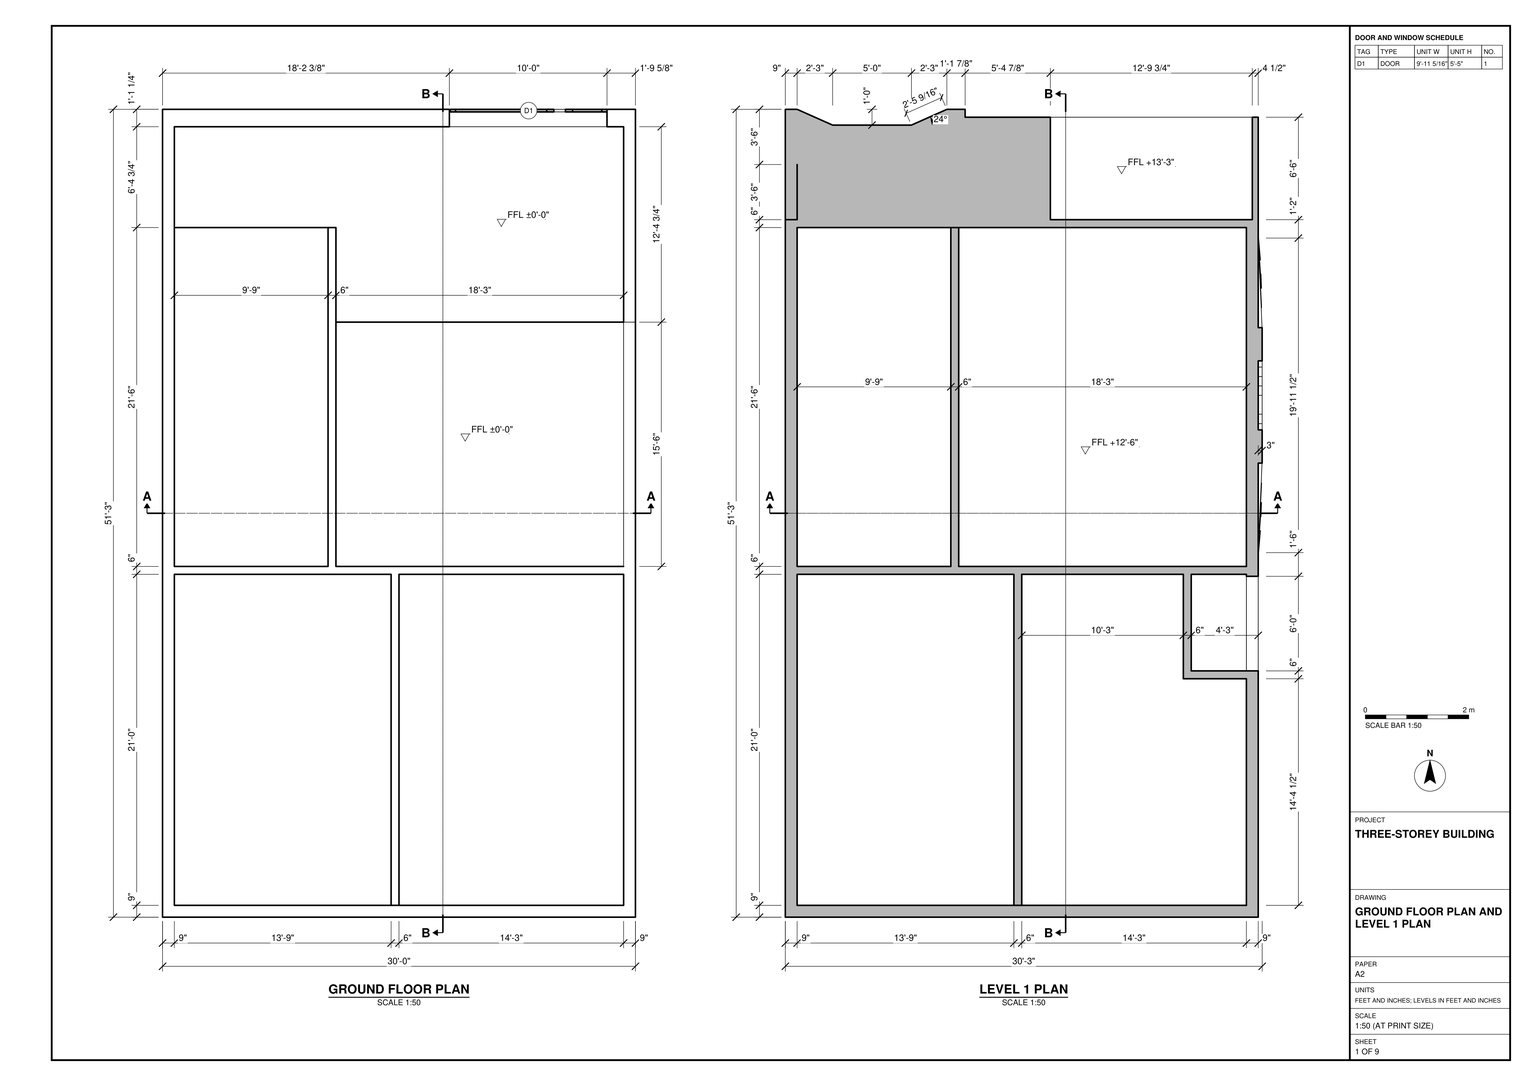
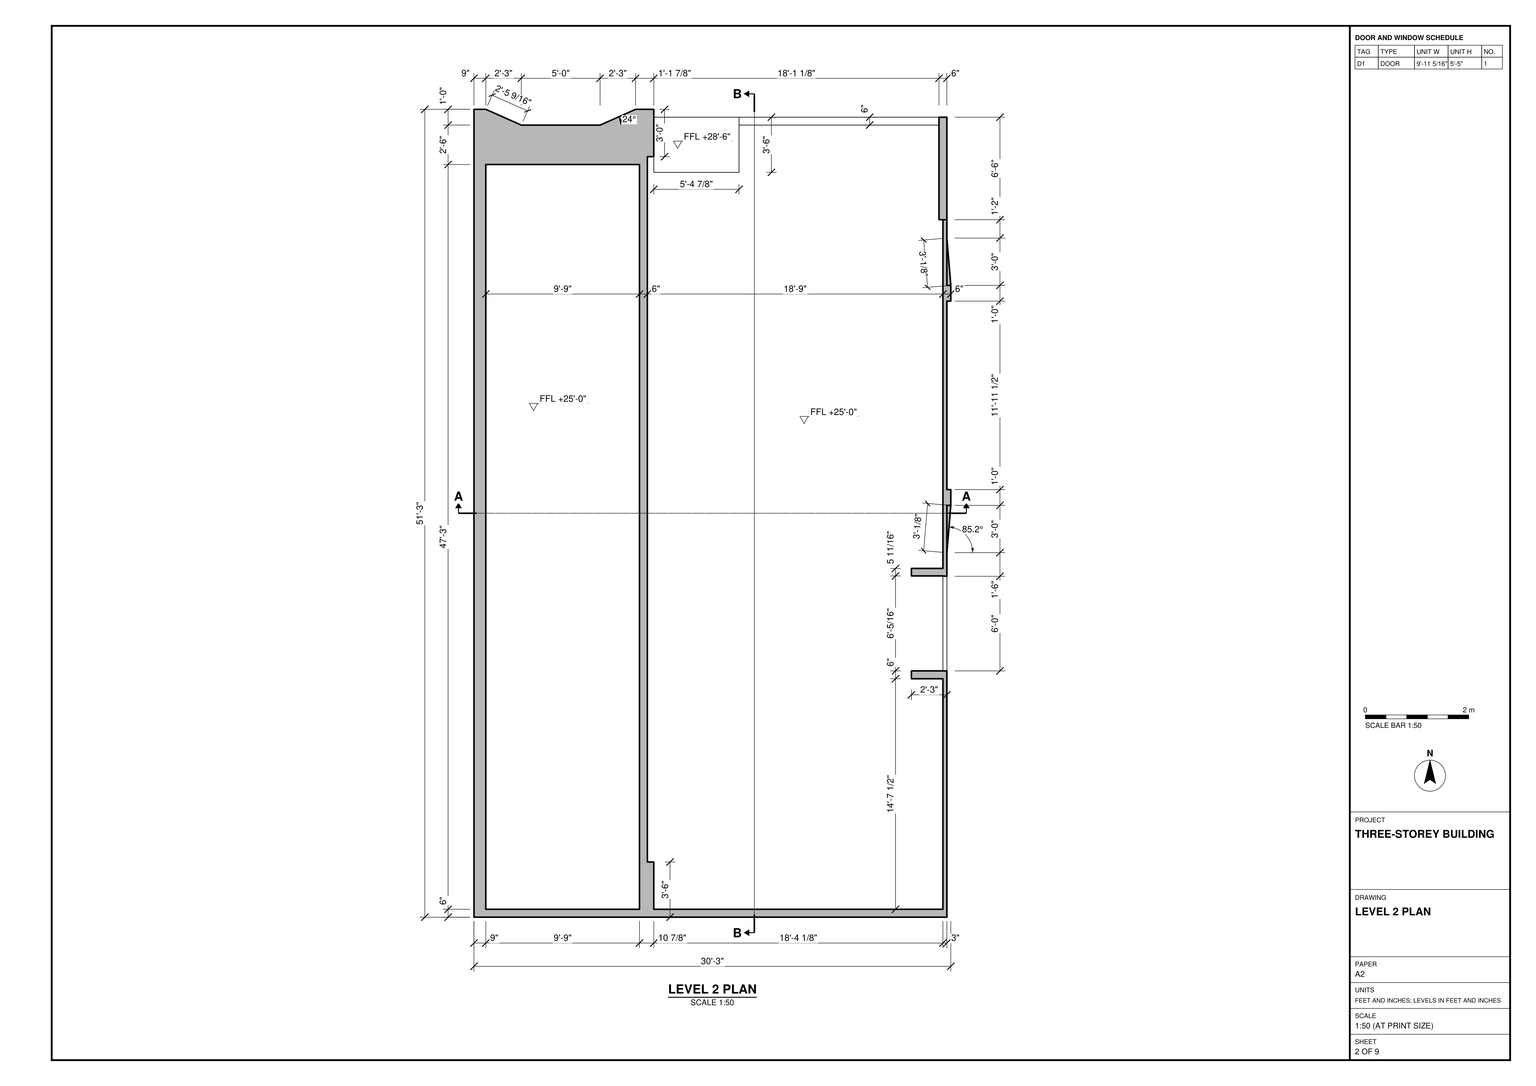
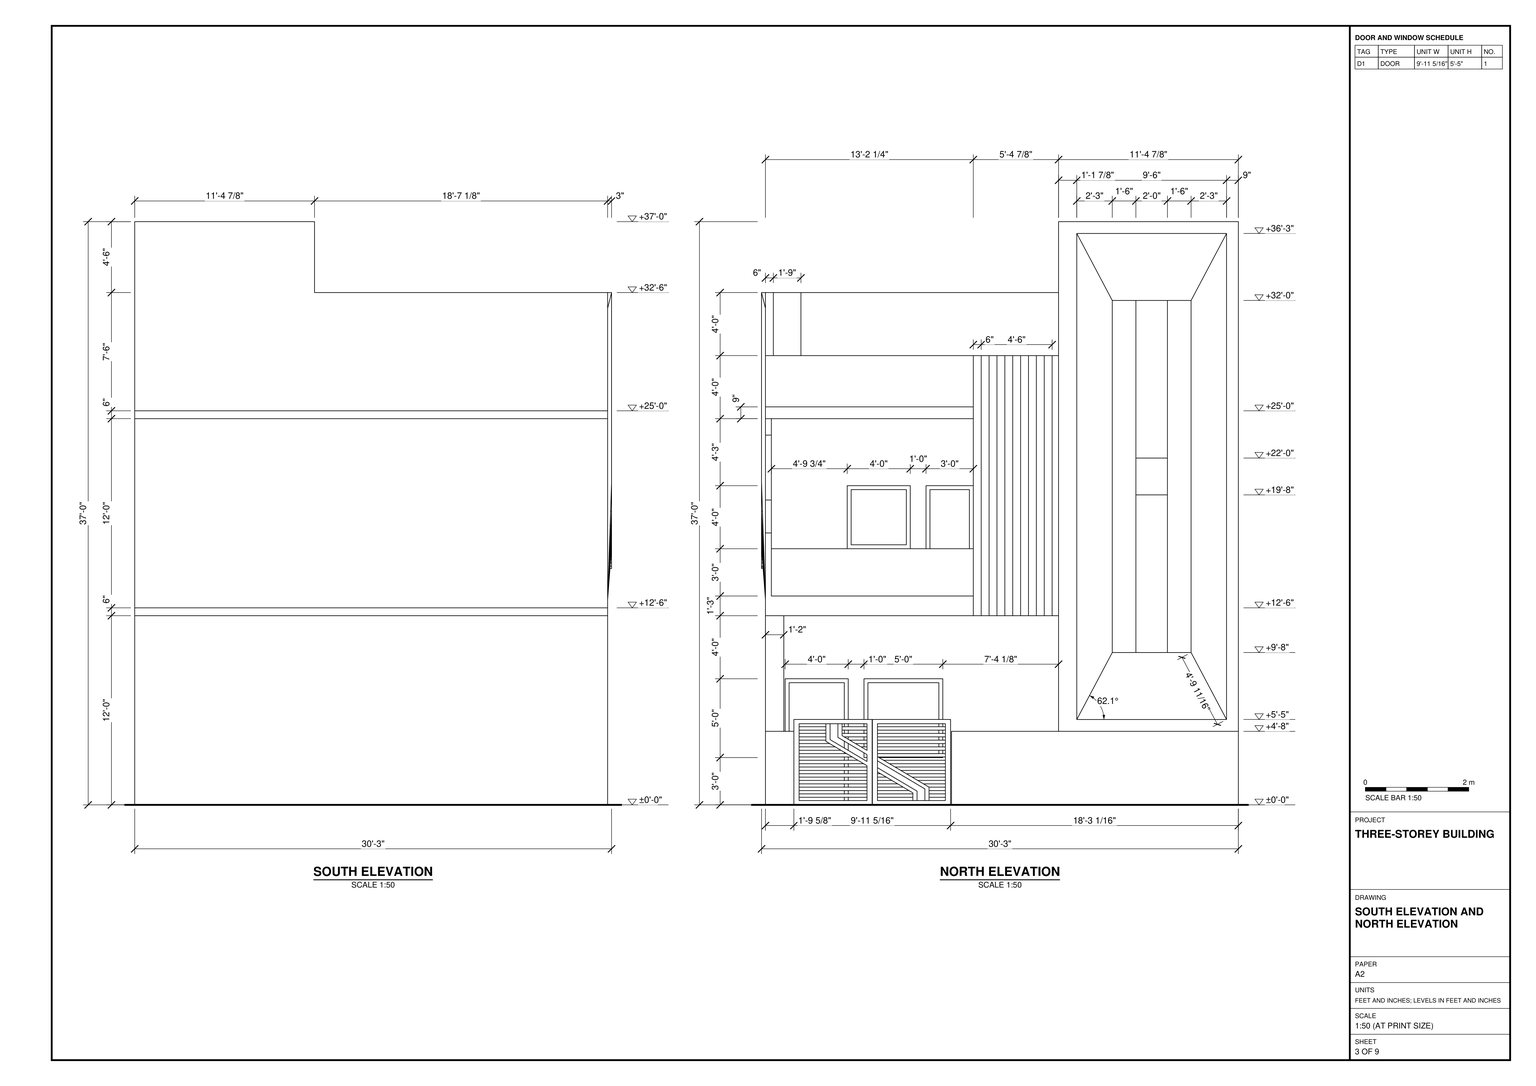
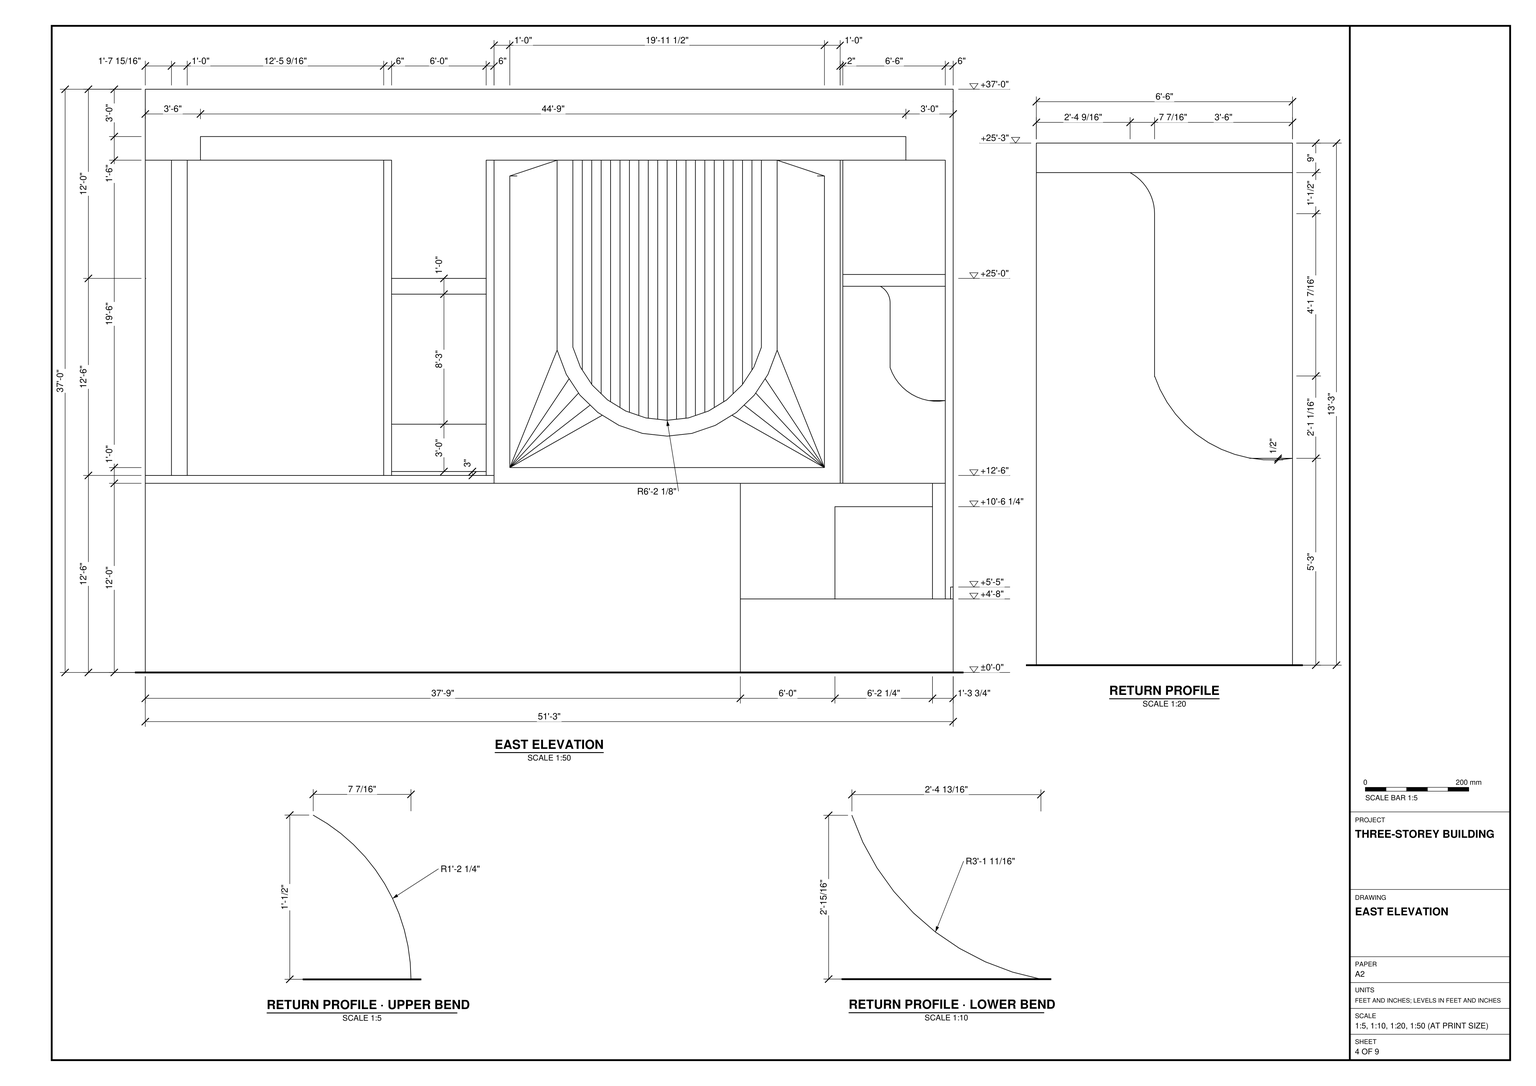
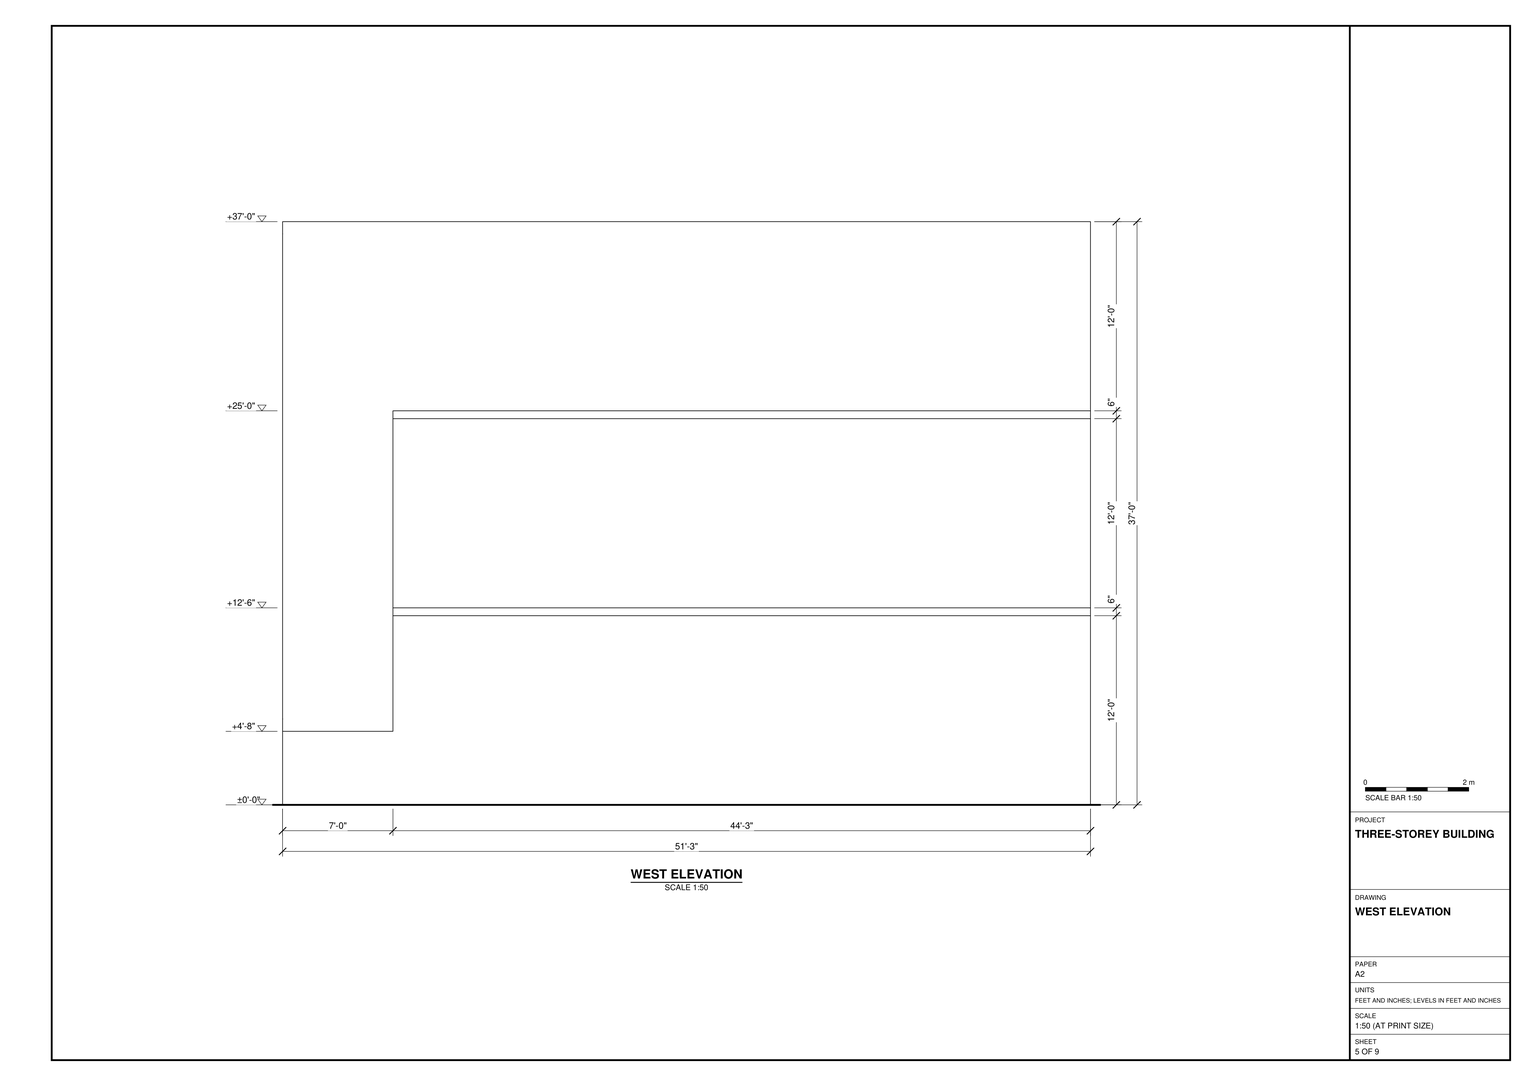
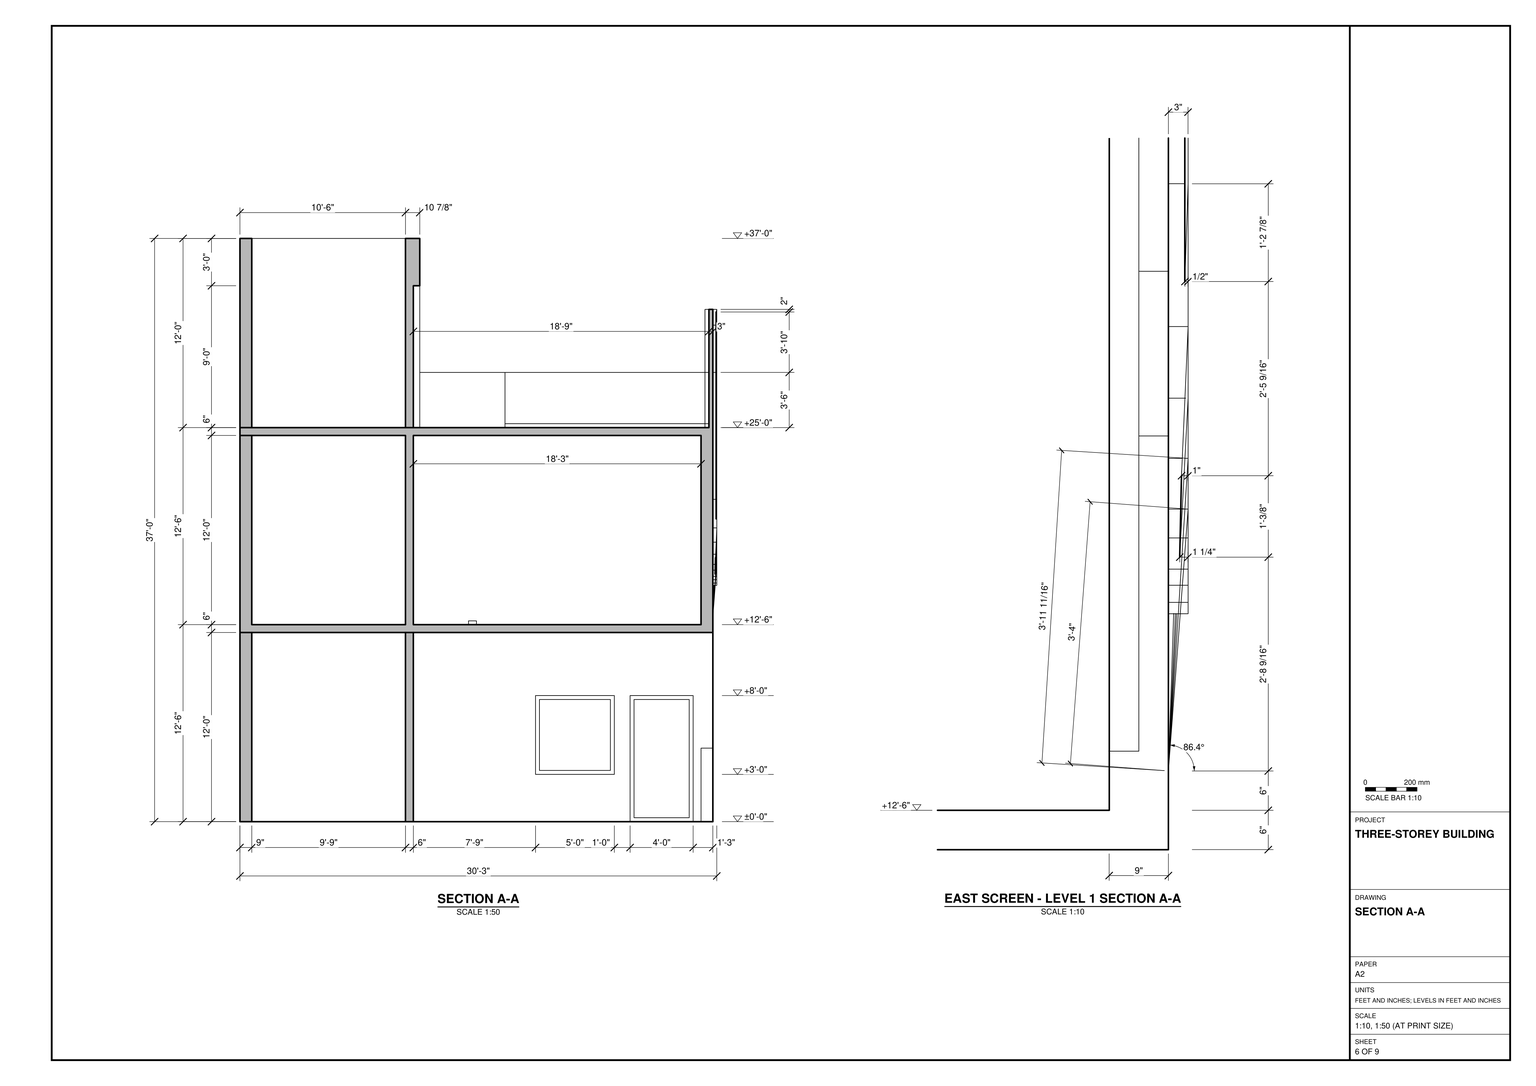
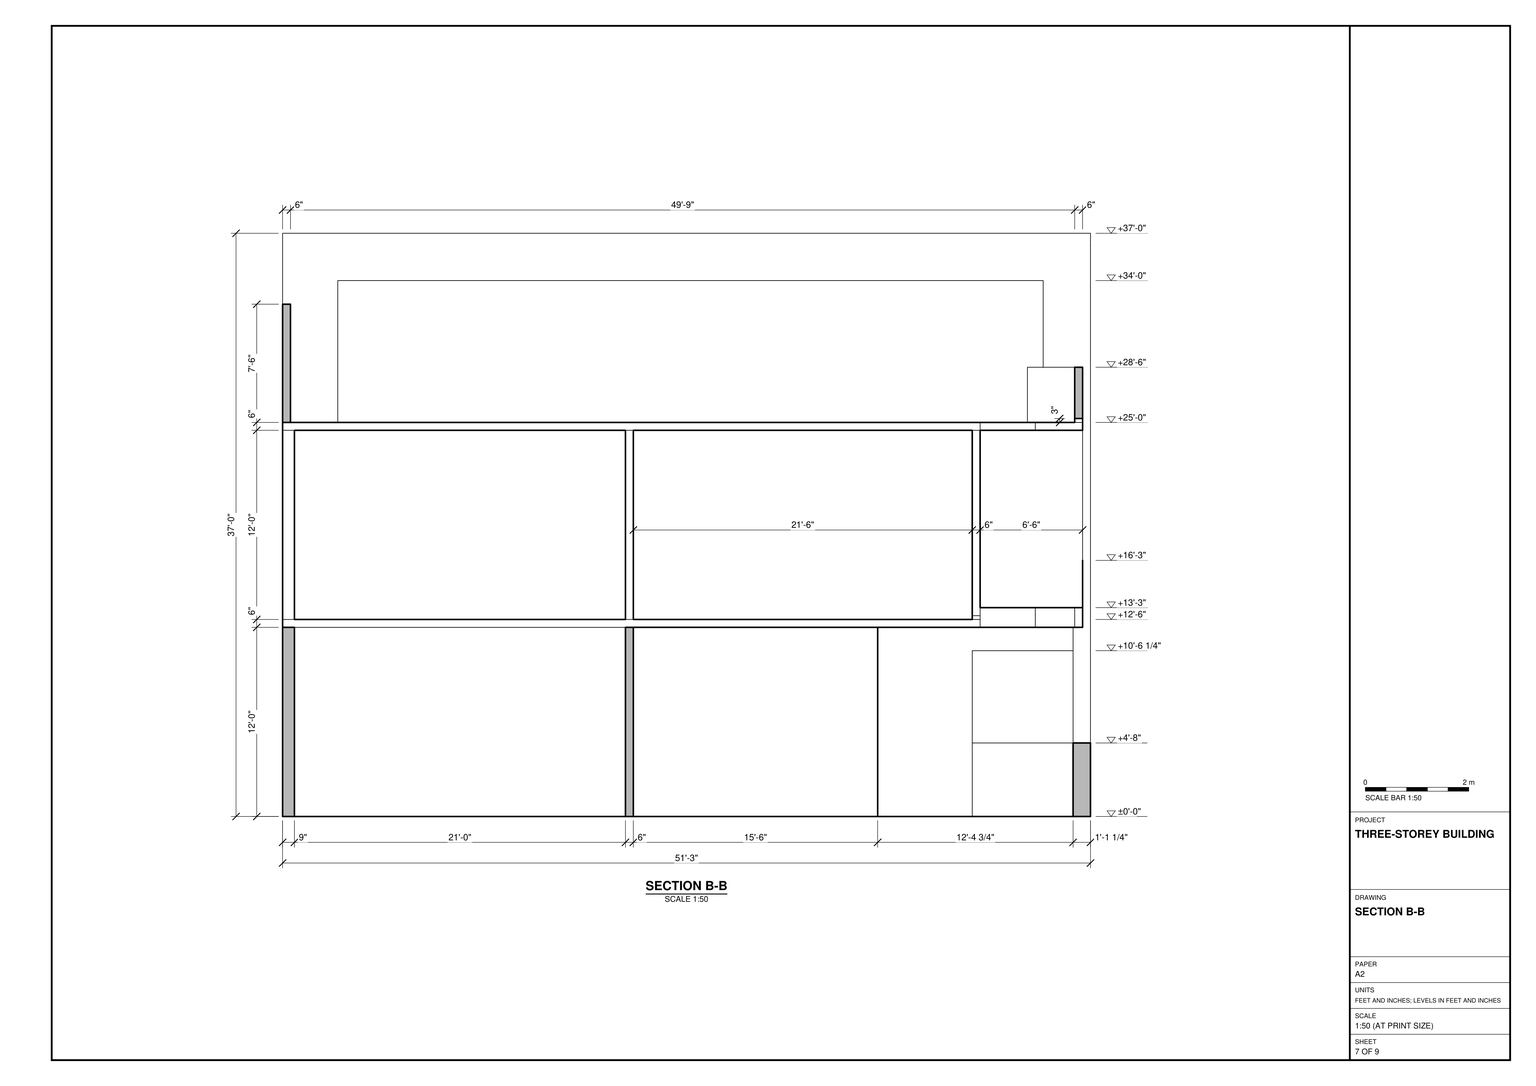
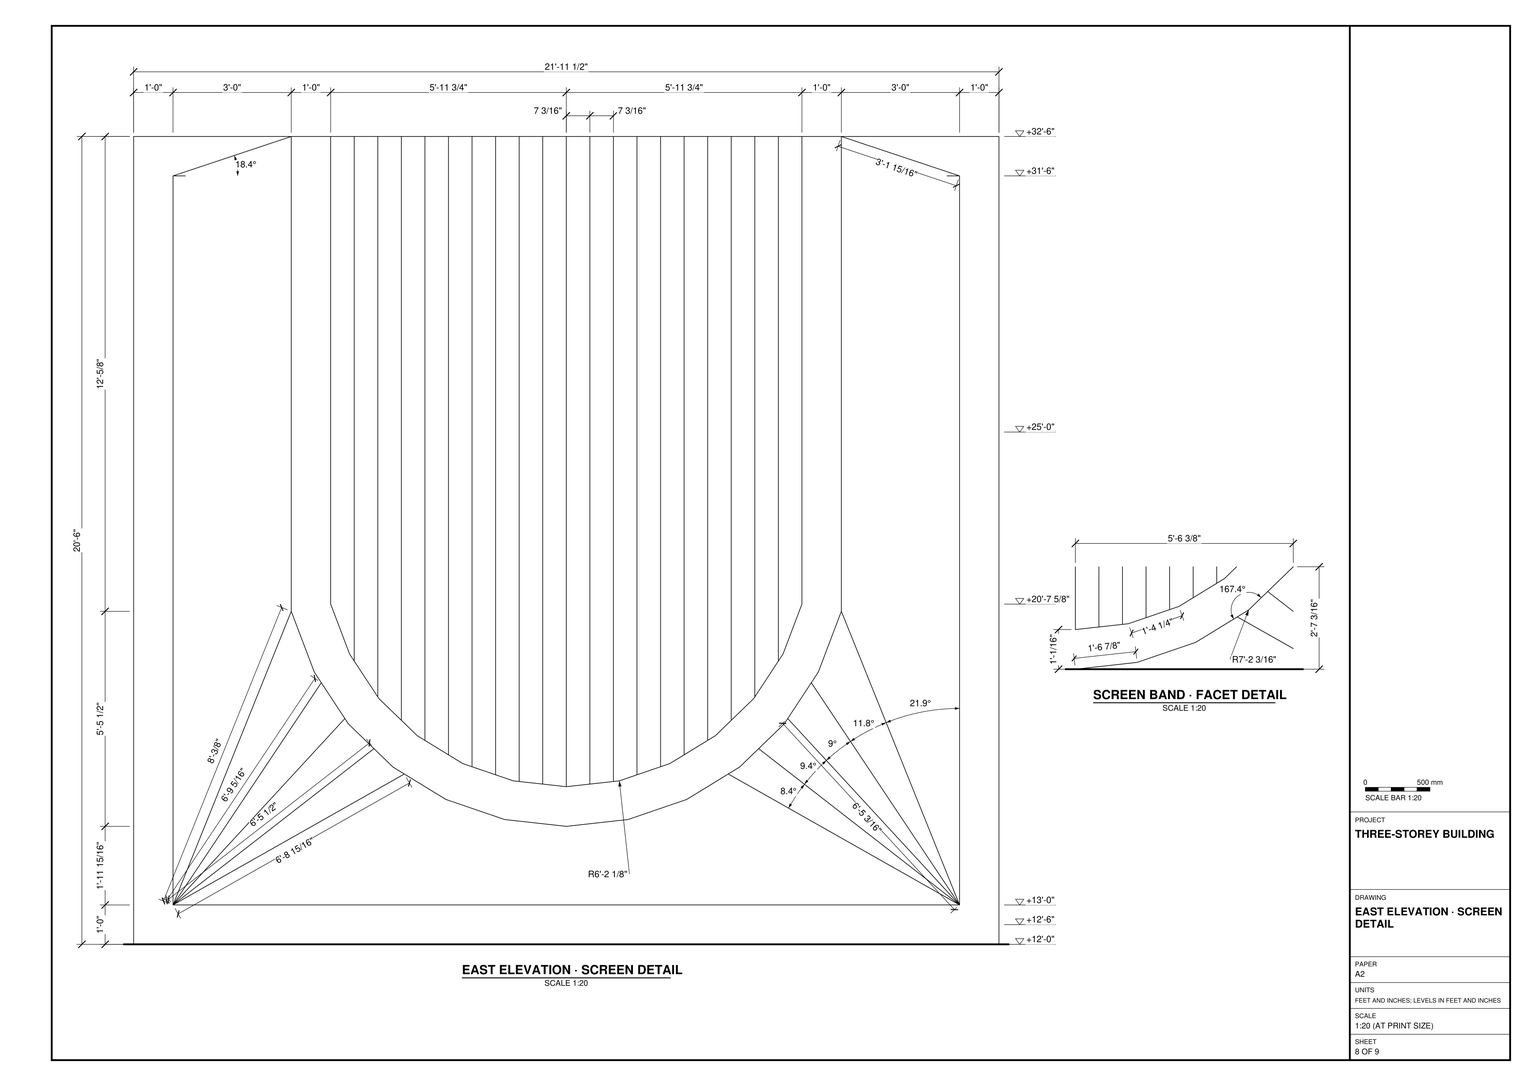
Work in feet and inches to build the three-storey building shown in task_files/diagram_01.pdf. The overall model measures 30'-3" east to west, 51'-3" north to south and 37'-0" high. Set the ground floor at ±0'-0", level 1 at +12'-6" and level 2 at +25'-0".

Use each floor plan separately: the partitions change between storeys. On the ground floor, place the two rear bays side by side and offset their dividing wall from the partition farther north. On level 1, follow the wall return on the east side. On level 2, form the long, narrow western bay beside the wider eastern area. Use the wall thicknesses shown, including the 9" perimeter walls and 6" partitions where indicated. Match the floor slabs and stepped roof edges to the elevations.

On the north frontage, place the two-leaf entrance gate in the low wall and set the window openings behind it. Model the vertical fins and the tall recessed panel with sloping reveals. Keep shell elements such as walls, slabs and roof separate as groups or components. Group each furniture or joinery piece shown separately and use components for repeated parts. Decor and loose items may be any suitable library components. Save one SketchUp model as output_files/three_storey_building_with_a_stepped_roofline.skp.

# SketchUp Ruby script. Lengths in inches.
U = 1.inch
M = Sketchup.active_model
def pt(a) = Geom::Point3d.new(a.map { |v| v * U })
def face(e, loops, mat)
  f = e.add_face(loops[0].map { |a| pt(a) })
  loops[1..].each { |l| e.add_face(l.map { |a| pt(a) }).erase! }
  f.material = f.back_material = mat if mat
  f
end
# faces: each face lists its corners as indices into pts; further lists are holes
def faces(e, pts, list, mat = nil) = list.each { |f| face(e, (f[0].is_a?(Array) ? f : [f]).map { |l| l.map { |i| pts[i] } }, mat) }
# xy, xz, yz: faces in a plane at the given z, y or x. An outline is a flat list of corners, or four numbers for a rectangle; further outlines are holes
def ring(l) = l.size == 4 ? [[l[0], l[1]], [l[2], l[1]], [l[2], l[3]], [l[0], l[3]]] : l.each_slice(2).to_a
def flat(e, list, mat, &to3) = list.each { |f| face(e, (f[0].is_a?(Array) ? f : [f]).map { |l| ring(l).map { |u, v| to3.(u, v) } }, mat) }
def xy(e, z, list, mat = nil) = flat(e, list, mat) { |x, y| [x, y, z] }
def xz(e, y, list, mat = nil) = flat(e, list, mat) { |x, z| [x, y, z] }
def yz(e, x, list, mat = nil) = flat(e, list, mat) { |y, z| [x, y, z] }
def lines(e, pts, list) = list.each { |a, b| e.add_line(pt(pts[a]), pt(pts[b])) }
# prism: a flat outline (further loops are holes) pulled along v
def prism(e, loops, v, mat = nil)
  f = face(e, loops, mat); d = Geom::Vector3d.new(v.map { |x| x * U })
  f.pushpull(f.normal.samedirection?(d) ? d.length : -d.length)
end
def box(e, o, s, mat = nil) = prism(e, [[o, [o[0] + s[0], o[1], o[2]], [o[0] + s[0], o[1] + s[1], o[2]], [o[0], o[1] + s[1], o[2]]]], [0, 0, s[2]], mat)
def at(x, y, z, deg = 0) = Geom::Transformation.translation(pt([x, y, z])) * Geom::Transformation.rotation(ORIGIN, Z_AXIS, deg.degrees)
def axes(o, x, y, z) = Geom::Transformation.new([*x, 0, *y, 0, *z, 0, *pt(o).to_a, 1])
def part(name) = M.definitions.add(name)
# library, detail: a bought-in or finely detailed component or shape, given as its bounding box
def library(name, o, s) = part(name).tap { |d| box(d.entities, o, s) }
def detail(e, o, s) = box(e.add_group.entities, o, s)
def put(e, d, t, mat = nil) = e.add_instance(d, t).tap { |i| i.material = mat if mat }
def group(e, t, mat = nil) = e.add_group.tap { |g| g.transformation = t; g.material = mat if mat }.entities
root = M.entities
M.materials.add("B03_Apricot_Glow").color = [255, 140, 101]
M.materials.add("Carpet_2_1K").color = [173, 65, 48]
M.materials.add("Crushed_Rock_Gravel_1K").color = [234, 234, 234]
M.materials.add("Glass_Basic_01").color = [149, 186, 85]
M.materials["Glass_Basic_01"].alpha = 0.25
M.materials.add("Glass_Mirror_01").color = [185, 185, 185]
M.materials.add("ThomThom - Trousers1").color = [162, 168, 168]
M.materials.add("ThomThom - Waistcoat2").color = [127, 127, 126]
M.materials.add("Wood_Veneer_15_1K").color = [103, 69, 45]
c1 = library("Modern+Gate+1",[0,0,0],[118.11,1.97,78.74])
xy(root,0,[[[0,0,360,0,360,453,351,453,351,267,132,267,132,525,126,525,126,267,9,267,9,601.76,218.36,601.76,218.36,615,0,615],[180,9,351,261],[9,9,174,261]],[9,9,174,261],[180,9,351,261],[9,267,126,525],[132,267,351,453],
  [132,453,351,453,351,601.76,9,601.76,9,525,132,525],[351,453,360,453,360,615,338.36,615,338.36,601.76,351,601.76],[218.36,601.76,338.36,615]])
xy(root,55.98,[[351,453,360,599.24],[346.02,599.24,351,601.76],[351,599.24,351,601.76,346.02,601.76,346.02,609,360,609,360,599.24],[136.89,601.76,218.36,615],[338.36,601.76,346.02,601.76,346.02,609,360,609,360,615,338.36,615]])
xy(root,126.22,[[126,525,132,601.76]])
xy(root,144,[[0,0,9,531],[[9,0,9,9,174,9,174,261,132,261,132,267,351,267,351,453,360,453,360,0],[180,9,351,261]],[[9,9,9,525,126,525,126,601.76,132,601.76,132,453,351,453,351,267,132,267,132,261,174,261,174,9],[126,348,132,354]],[9,261,132,261,132,348,126,348,126,267,9,267],[126,348,132,354],
  [126,354,132,601.76],[9,525,126,601.76],[346.02,599.24,360,609]])
xy(root,144,[[132,453,132,601.76,136.89,601.76,136.89,609,346.02,609,346.02,599.24,360,599.24,360,453]],"Wood_Veneer_15_1K")
xy(root,150,[[9,9,174,261],[180,9,351,9,351,181.5,303,181.5,303,261,180,261],[309,187.5,351,261],[9,267,126,525],[132,267,351,525]])
xy(root,153,[[351,187.5,360,259.5]])
xy(root,159,[[201.77,531,355.5,609]])
xy(root,207,[[355.5,596.6875,360,609]])
xy(root,288,[[303,181.5,351,181.5,351,187.5,309,187.5,309,261,303,261],[351,187.5,360,259.5]])
xy(root,294,[[0,0,0,531,9,531,9,525,351,525,351,267,132,267,132,525,126,525,126,267,9,267,9,261,174,261,174,9,9,9,9,0],[0,0,9,531],[180,9,351,261]])
xy(root,294,[[201.77,531,201.77,609,360,609,360,559.54,355.5,559.54,355.5,531]],"ThomThom - Trousers1")
xy(root,300,[[0,0,132,0,132,6,136.89,6,136.89,42,132,42,132,573,126,573,126,6,9,6,9,531,0,531],[132,0,360,0,354,6,132,6],[9,6,126,573],[136.89,6,357,6,357,181.5,333,181.5,333,187.5,357,187.5,357,259.79,333,259.79,333,265.5,357,265.5,357,531,354,531,354,603,201.77,603,201.77,567,136.89,567,136.89,579,132,579,132,42,136.89,42],[357,187.5,360,187.5,360,259.5,357,259.79],
  [132,579,136.89,603]])
xy(root,303,[[354,531,360,531,360,609,201.77,609,201.77,603,354,603]])
xy(root,342,[[132,603,136.89,609],[201.77,603,354,609]])
xy(root,342,[[136.89,567,201.77,609]],"B03_Apricot_Glow")
xy(root,390,[[136.89,0,360,0,360,181.5,357,181.5,357,6,136.89,6],[357,265.5,360,265.5,360,313.5,363,313.5,363,325.5,360,325.5,360,469,363,469,363,481,360,481,360,531,357,531],[354,531,360,609]])
xy(root,390,[[333,181.5,360,187.5],[360,259.5,360,265.5,333,265.5,333,259.79,357,259.79]],"ThomThom - Waistcoat2")
xy(root,408,[[132,42,136.89,579]])
xy(root,444,[[[0,0,136.89,615],[9,6,126,573]]])
xz(root,0,[[0,0,360,144],[0,144,360,150],[0,150,360,294],[0,294,360,300],[0,300,360,300,360,390,136.89,390,136.89,444,0,444]])
xz(root,6,[[9,300,126,444],[136.89,300,357,390]])
xz(root,9,[[9,0,174,144],[174,0,180,2.88],[180,0,351,144],[174,2.88,180,144],[9,150,174,294],
  [174,150,180,152.88],[180,150,351,294],[174,152.88,180,294]])
xz(root,42,[[132,300,136.89,408]])
xz(root,181.5,[[303,150,351,153],[303,153,351,288]])
xz(root,181.5,[[333,300,357,390]],"Glass_Basic_01")
xz(root,187.5,[[309,150,309,288,360,288,360,153,351,153,351,150],[333,300,360,390]],"ThomThom - Waistcoat2")
xz(root,259.5,[[351,153,360,288]],"ThomThom - Trousers1")
xz(root,259.79,[[333,300,357,390]],"ThomThom - Waistcoat2")
xz(root,261,[[9,0,174,144],[180,0,351,144],[9,150,174,294]])
xz(root,261,[[180,150,303,150,303,288,309,288,309,150,351,150,351,294,180,294]],"ThomThom - Waistcoat2")
xz(root,265.5,[[333,300,357,390]],"ThomThom - Waistcoat2")
xz(root,267,[[9,0,126,144],[132,0,351,144],[9,150,126,294],[132,150,351,294]])
xz(root,313.5,[[360,245.41,363,342],[360,342,363,378],[360,378,363,390]])
xz(root,325.5,[[360,247.6,363,342],[360,342,363,390]])
xz(root,453,[[[132,0,132,144,360,144,360,55.98,351,55.98,351,0,345,0,345,96,297,96,297,0],[225,36,285,96]]])
xz(root,453,[[228,39,282,93]],"Glass_Mirror_01")
xz(root,453,[[[297,0,345,96],[300,3,342,93]],[300,3,342,93],[[225,36,285,96],[228,39,282,93]]],"Wood_Veneer_15_1K")
xz(root,469,[[360,247.6,363,342],[360,342,363,390]])
xz(root,481,[[360,245.41,363,342],[360,342,363,378],[360,378,363,390]])
xz(root,525,[[9,0,126,144],[126,0,132,126.22],[9,150,126,294],[126,150,132,294],[132,150,174,150,174,152.88,180,152.88,180,150,351,150,351,294,132,294],
  [174,150,180,152.88]])
xz(root,531,[[0,144,9,150],[0,150,9,294],[[237.77,159,237.77,243,201.77,243,201.77,294,355.5,294,355.5,159],[249.77,195,297.77,243]],[0,294,9,300],[357,303,360,342],
  [354,342,357,390],[357,342,360,390]])
xz(root,531,[[354,300,357,303],[354,303,357,342]],"Glass_Basic_01")
xz(root,531,[[252.77,198,294.77,240]],"Glass_Mirror_01")
xz(root,531,[[[201.77,159,237.77,243],[204.77,162,234.77,240]],[204.77,162,234.77,240],[[249.77,195,297.77,243],[252.77,198,294.77,240]]],"Wood_Veneer_15_1K")
xz(root,567,[[355.5,232.07,360,281.49]])
xz(root,567,[[136.89,300,201.77,342]],"B03_Apricot_Glow")
xz(root,573,[[9,294,132,300],[9,300,126,444]])
xz(root,579,[[132,300,136.89,408]])
xz(root,599.24,[[346.02,55.98,360,144]],"ThomThom - Waistcoat2")
xz(root,601.76,[[9,0,218.36,55.98],[338.36,0,345,55.98],[345,0,351,55.98],[9,55.98,136.89,55.98,136.89,126.22,126,126.22,126,144,9,144],[132,126.22,136.89,144]])
xz(root,603,[[54,235.98,78,264],[132,300,136.89,342]])
xz(root,603,[[36,115.98,54,384],[78,115.98,96,384]],"Carpet_2_1K")
xz(root,603,[[201.77,300,354,303],[201.77,303,354,342]],"Glass_Basic_01")
xz(root,603,[[54,115.98,78,235.98],[54,264,78,384]],"Glass_Mirror_01")
xz(root,609,[[201.77,144,201.77,159,355.5,159,355.5,207,360,207,360,144],[132,294,136.89,300],[132,300,136.89,342],[354,342,360,390]])
xz(root,609,[[136.89,144,141.77,342],[141.77,144,147.77,342],[147.77,144,153.77,342],[153.77,144,159.77,342],[159.77,144,165.77,342],
  [165.77,144,171.77,342],[171.77,144,177.77,342],[177.77,144,183.77,342],[183.77,144,189.77,342],[189.77,144,195.77,342],
  [195.77,144,201.77,342]],"B03_Apricot_Glow")
xz(root,609,[[201.77,159,355.5,195],[201.77,303,360,342]],"Glass_Basic_01")
xz(root,609,[[201.77,294,360,303]],"ThomThom - Trousers1")
xz(root,609,[[346.02,55.98,360,144]],"ThomThom - Waistcoat2")
xz(root,615,[[0,0,218.36,55.98],[[0,55.98,136.89,444],[9,64.98,123,435]]])
xz(root,615,[[338.36,0,360,55.98]],"B03_Apricot_Glow")
yz(root,0,[[0,0,0,144,531,144,531,55.98,615,55.98,615,0],[531,55.98,531,300,0,300,0,444,615,444,615,55.98],[0,144,531,150],[0,150,531,294],[0,294,531,300]])
yz(root,9,[[9,0,261,144],[267,0,525,144],[525,0,601.76,55.98],[525,55.98,601.76,144],[531,144,573,294],
  [9,150,261,294],[267,150,525,294],[531,294,573,300],[6,300,573,444]])
yz(root,126,[[267,0,525,144],[525,126.22,601.76,144],[267,150,525,294],[6,300,573,444]])
yz(root,132,[[267,0,453,144],[453,0,525,0,525,126.22,601.76,126.22,601.76,144,453,144],[267,150,525,294],[573,294,609,300],[42,300,579,408],
  [603,300,609,342]])
yz(root,136.89,[[601.76,55.98,615,55.98,615,444,0,444,0,390,6,390,6,300,42,300,42,408,579,408,579,342,609,342,609,144,601.76,144],[567,300,579,342],[579,300,603,342]])
yz(root,174,[[9,0,261,144],[9,150,261,294]])
yz(root,180,[[9,0,261,144],[9,150,261,294]])
yz(root,201.77,[[603,300,609,303]])
yz(root,201.77,[[531,159,609,294],[567,300,603,342],[603,303,609,342]],"B03_Apricot_Glow")
yz(root,218.36,[[601.76,0,615,55.98]])
yz(root,303,[[181.5,150,261,288]])
yz(root,309,[[187.5,150,261,288]],"ThomThom - Waistcoat2")
yz(root,333,[[259.79,300,265.5,390]])
yz(root,333,[[181.5,300,187.5,390]],"Glass_Basic_01")
yz(root,338.36,[[601.76,0,615,55.98]])
yz(root,346.02,[[599.24,55.98,609,144]],"ThomThom - Waistcoat2")
yz(root,351,[[9,0,261,144],[453,0,601.76,55.98],[9,150,9,294,187.5,294,187.5,288,181.5,288,181.5,150],[187.5,150,187.5,153,259.5,153,259.5,294,261,294,261,150],[267,150,525,294],
  [187.5,288,259.5,294]])
yz(root,354,[[531,342,609,390]])
yz(root,354,[[531,300,603,303],[531,303,603,342]],"Glass_Basic_01")
yz(root,355.5,[[531,159,609,207],[531,207,531,294,559.54,294,560.64,293.34,561.67,292.59,562.625,291.75,563.5,290.83,564.29,289.84,564.99,288.77,565.6,287.65,566.1,286.48,566.49,285.27,566.77,284.02,566.94,282.76,567,281.49,567,207],[567,207,567,232.07,568.67,227.96,570.81,224.08,573.39,220.47,576.37,217.2,579.72,214.29,583.38,211.8,587.32,209.76,591.46,208.1875,595.76,207.12,596.6875,207]])
yz(root,357,[[6,300,181.5,390],[265.5,300,531,390]],"Glass_Basic_01")
yz(root,360,[[0,0,453,144],[453,0,615,55.98],[0,144,265.5,150],[265.5,144,529,144,529,390,481,390,481,378,517,378,517,156,277.5,156,277.5,378,313.5,378,313.5,390,265.5,390],[529,144,531,390],
  [0,150,19.93,390],[187.5,150,259.5,153],[277.5,156,517,156,517,378,481,378,481,245.41,474,226.92,471.85,223.66,464.68,212.75,463.61,211.13,455.82,203.59,450.03,197.99,446.57,195.86,439.39,191.47,433.92,188.12,429.83,186.72,422.66,184.27,416.03,182,412.92,181.66,405.74,180.86,397.25,179.93,381.58,181.66,378.47,182,371.84,184.27,364.67,186.72,360.58,188.12,355.11,191.47,347.93,195.86,344.47,197.99,338.68,203.59,330.89,211.13,329.82,212.75,322.65,223.66,320.5,226.92,313.5,245.41,313.5,378,277.5,378],[604.59,206.52,609,207,596.6875,207,600.16,206.56]])
yz(root,360,[[397.25,192,397.25,390,390.08,390,390.08,192.79],[397.25,192,404.42,192.79,404.42,390,397.25,390],[390.08,192.79,390.08,390,382.9,390,382.9,193.58],[404.42,192.79,411.6,193.58,411.6,390,404.42,390],[382.9,193.58,382.9,390,375.72,390,375.72,195.62,381.1,193.78],
  [411.6,193.58,413.4,193.78,418.78,195.62,418.78,390,411.6,390],[375.72,195.62,375.72,390,368.55,390,368.55,198.07],[418.78,195.62,425.95,198.07,425.95,390,418.78,390],[368.55,198.07,368.55,390,361.375,390,361.375,201.7,365.72,199.04],[425.95,198.07,428.78,199.04,433.125,201.7,433.125,390,425.95,390],
  [361.375,201.7,361.375,390,354.2,390,354.2,206.1],[433.125,201.7,440.3,206.1,440.3,390,433.125,390],[354.2,206.1,354.2,390,347.03,390,347.03,212.21,351.86,207.53],[440.3,206.1,442.64,207.53,447.48,212.21,447.48,390,440.3,390],[347.03,212.21,347.03,390,339.85,390,339.85,219.34,340.1875,218.83],
  [447.48,212.21,454.3125,218.83,454.65,219.34,454.65,390,447.48,390],[339.85,219.34,339.85,390,332.67,390,332.67,230.25],[454.65,219.34,461.83,230.25,461.83,390,454.65,390],[332.67,230.25,332.67,390,325.5,390,325.5,247.6,331.26,232.41],[461.83,230.25,463.24,232.41,469,247.6,469,390,461.83,390]],"B03_Apricot_Glow")
yz(root,360,[[31.93,150,181.5,390]],"Crushed_Rock_Gravel_1K")
yz(root,360,[[531,144,609,144,609,207,604.59,206.52,600.16,206.56,596.6875,207,595.76,207.12,591.46,208.1875,587.32,209.76,583.38,211.8,579.72,214.29,576.37,217.2,573.39,220.47,570.81,224.08,568.67,227.96,567,232.07,567,281.49,566.94,282.76,566.77,284.02,566.49,285.27,566.1,286.48,565.6,287.65,564.99,288.77,564.29,289.84,563.5,290.83,562.625,291.75,561.67,292.59,560.64,293.34,559.54,294,531,294],[187.5,153,259.5,189],[531,303,609,390]],"Glass_Basic_01")
yz(root,360,[[531,294,609,303]],"ThomThom - Trousers1")
yz(root,360,[[599.24,55.98,609,144],[19.93,150,31.93,390],[181.5,150,187.5,390],[259.5,150,265.5,390],[187.5,288,259.5,300]],"ThomThom - Waistcoat2")
yz(root,363,[[397.25,179.93,405.74,180.86,412.92,181.66,416.03,182,422.66,184.27,429.83,186.72,433.92,188.12,439.39,191.47,446.57,195.86,450.03,197.99,455.82,203.59,463.61,211.13,464.68,212.75,471.85,223.66,474,226.92,481,245.41,481,390,469,390,469,247.6,463.24,232.41,461.83,230.25,454.65,219.34,454.3125,218.83,447.48,212.21,442.64,207.53,440.3,206.1,433.125,201.7,428.78,199.04,425.95,198.07,418.78,195.62,413.4,193.78,411.6,193.58,404.42,192.79,397.25,192,382.9,193.58,381.1,193.78,375.72,195.62,368.55,198.07,365.72,199.04,361.375,201.7,354.2,206.1,351.86,207.53,347.03,212.21,340.1875,218.83,339.85,219.34,332.67,230.25,331.26,232.41,325.5,247.6,325.5,390,313.5,390,313.5,245.41,320.5,226.92,322.65,223.66,329.82,212.75,330.89,211.13,338.68,203.59,344.47,197.99,347.93,195.86,355.11,191.47,360.58,188.12,364.67,186.72,371.84,184.27,378.47,182,381.58,181.66]])
p = [[36,603,115.98],[9,615,64.98],[9,615,435],[36,603,384],[54,603,115.98],[78,603,115.98],
  [96,603,115.98],[123,615,64.98],[96,603,384],[123,615,435],[363,313.5,390],[360,277.5,378],
  [360,277.5,342],[360,277.5,303],[360,277.5,294],[360,277.5,156],[363,313.5,245.41],[363,313.5,342],
  [363,313.5,378],[363,329.82,212.75],[363,322.65,223.66],[360,517,156],[363,471.85,223.66],[363,464.68,212.75],
  [363,481,245.41],[360,517,303],[360,517,342],[360,517,378],[363,481,390],[363,481,378],
  [363,481,342],[360,381.58,181.66],[360,397.25,179.93],[363,397.25,179.93],[363,381.58,181.66],[360,405.74,180.86],
  [363,405.74,180.86],[360,412.92,181.66],[363,412.92,181.66],[360,378.47,182],[363,378.47,182],[360,416.03,182],
  [363,416.03,182],[360,371.84,184.27],[363,371.84,184.27],[360,422.66,184.27],[363,422.66,184.27],[360,364.67,186.72],
  [363,364.67,186.72],[360,429.83,186.72],[363,429.83,186.72],[360,360.58,188.12],[363,360.58,188.12],[360,433.92,188.12],
  [363,433.92,188.12],[360,355.11,191.47],[363,355.11,191.47],[360,439.39,191.47],[363,439.39,191.47],[360,347.93,195.86],
  [363,347.93,195.86],[360,446.57,195.86],[363,446.57,195.86],[360,390.08,192.79],[360,382.9,193.58],[363,382.9,193.58],
  [363,397.25,192],[360,397.25,192],[360,404.42,192.79],[363,404.42,192.79],[360,411.6,193.58],[363,411.6,193.58],
  [360,381.1,193.78],[363,381.1,193.78],[360,413.4,193.78],[363,413.4,193.78],[360,375.72,195.62],[363,375.72,195.62],
  [360,418.78,195.62],[363,418.78,195.62],[360,368.55,198.07],[363,368.55,198.07],[360,425.95,198.07],[363,425.95,198.07],
  [360,344.47,197.99],[363,344.47,197.99],[360,450.03,197.99],[363,450.03,197.99],[360,338.68,203.59],[363,338.68,203.59],
  [360,455.82,203.59],[363,455.82,203.59],[360,365.72,199.04],[363,365.72,199.04],[360,428.78,199.04],[363,428.78,199.04],
  [360,361.375,201.7],[363,361.375,201.7],[360,433.125,201.7],[363,433.125,201.7],[360,354.2,206.1],[363,354.2,206.1],
  [360,440.3,206.1],[363,440.3,206.1],[360,330.89,211.13],[363,330.89,211.13],[360,463.61,211.13],[363,463.61,211.13],
  [360,351.86,207.53],[363,351.86,207.53],[360,442.64,207.53],[363,442.64,207.53],[360,595.76,207.12],[360,596.6875,207],
  [355.5,596.6875,207],[355.5,595.76,207.12],[360,591.46,208.1875],[355.5,591.46,208.1875],[360,347.03,212.21],[363,347.03,212.21],
  [360,447.48,212.21],[363,447.48,212.21],[360,587.32,209.76],[355.5,587.32,209.76],[360,583.38,211.8],[355.5,583.38,211.8],
  [360,329.82,212.75],[360,464.68,212.75],[360,579.72,214.29],[355.5,579.72,214.29],[360,340.1875,218.83],[363,340.1875,218.83],
  [360,454.3125,218.83],[363,454.3125,218.83],[360,322.65,223.66],[360,471.85,223.66],[360,576.37,217.2],[355.5,576.37,217.2],
  [360,573.39,220.47],[355.5,573.39,220.47],[360,339.85,219.34],[363,339.85,219.34],[360,454.65,219.34],[363,454.65,219.34],
  [360,332.67,230.25],[363,332.67,230.25],[360,461.83,230.25],[363,461.83,230.25],[360,570.81,224.08],[355.5,570.81,224.08],
  [360,320.5,226.92],[363,320.5,226.92],[360,474,226.92],[363,474,226.92],[360,568.67,227.96],[355.5,568.67,227.96],
  [360,313.5,245.41],[360,481,245.41],[360,567,232.07],[355.5,567,232.07],[360,331.26,232.41],[363,331.26,232.41],
  [360,463.24,232.41],[363,463.24,232.41],[360,325.5,247.6],[363,325.5,247.6],[360,469,247.6],[363,469,247.6],
  [360,566.94,282.76],[360,567,281.49],[355.5,567,281.49],[355.5,566.94,282.76],[360,566.77,284.02],[355.5,566.77,284.02],
  [360,566.49,285.27],[355.5,566.49,285.27],[360,566.1,286.48],[355.5,566.1,286.48],[360,565.6,287.65],[355.5,565.6,287.65],
  [360,564.99,288.77],[355.5,564.99,288.77],[360,564.29,289.84],[355.5,564.29,289.84],[360,563.5,290.83],[355.5,563.5,290.83],
  [360,562.625,291.75],[355.5,562.625,291.75],[360,561.67,292.59],[355.5,561.67,292.59],[360,560.64,293.34],[355.5,560.64,293.34],
  [360,559.54,294],[355.5,559.54,294],[357,259.79,300],[360,259.5,300],[360,259.5,390],[357,259.79,390],
  [78,603,384],[54,603,384],[180,525,152.88],[180,531,152.88],[180,525,150],[180,531,150],
  [360,567,207],[355.5,567,207],[132,573,150],[132,573,294]]
faces(root,p,[[0,1,2,3],[1,0,4,5,6,7],[7,6,8,9],[10,11,12,13,14,15,16,17,18],[15,19,20],[21,22,23],[24,21,25,26,27,28,29,30],[31,32,33,34],
  [32,35,36,33],[35,37,38,36],[39,31,34,40],[37,41,42,38],[43,39,40,44],[41,45,46,42],[47,43,44,48],[45,49,50,46],
  [51,47,48,52],[49,53,54,50],[55,51,52,56],[53,57,58,54],[59,55,56,60],[57,61,62,58],[63,64,65,66,67],[68,67,66,69],
  [70,68,69,71],[64,72,73,65],[74,70,71,75],[72,76,77,73],[78,74,75,79],[76,80,81,77],[82,78,79,83],[84,59,60,85],
  [61,86,87,62],[88,84,85,89],[86,90,91,87],[80,92,93,81],[94,82,83,95],[92,96,97,93],[98,94,95,99],[96,100,101,97],
  [102,98,99,103],[104,88,89,105],[90,106,107,91],[100,108,109,101],[110,102,103,111],[112,113,114,115],[116,112,115,117],[108,118,119,109],
  [120,110,111,121],[122,116,117,123],[124,122,123,125],[126,104,105,19],[106,127,23,107],[128,124,125,129],[118,130,131,119],[132,120,121,133],
  [134,126,19,20],[127,135,22,23],[136,128,129,137],[138,136,137,139],[130,140,141,131],[142,132,133,143],[140,144,145,141],[146,142,143,147],
  [148,138,139,149],[150,134,20,151],[135,152,153,22],[154,148,149,155],[156,150,151,16],[152,157,24,153],[158,154,155,159],[144,160,161,145],
  [162,146,147,163],[160,164,165,161],[166,162,163,167],[168,169,170,171],[172,168,171,173],[174,172,173,175],[176,174,175,177],[178,176,177,179],
  [180,178,179,181],[182,180,181,183],[184,182,183,185],[186,184,185,187],[188,186,187,189],[190,188,189,191],[192,190,191,193],[9,8,198,199,3,2]])
faces(root,p,[[194,195,196,197]],"ThomThom - Trousers1")
lines(root,p,[[200,201],[202,203],[204,205],[206,207],[62,21],[21,91],[89,15],[60,15]])
put(root,c1,axes([219.07,613.03,0],[1.01,0,0],[0,1,0],[0,0,0.82586]))
